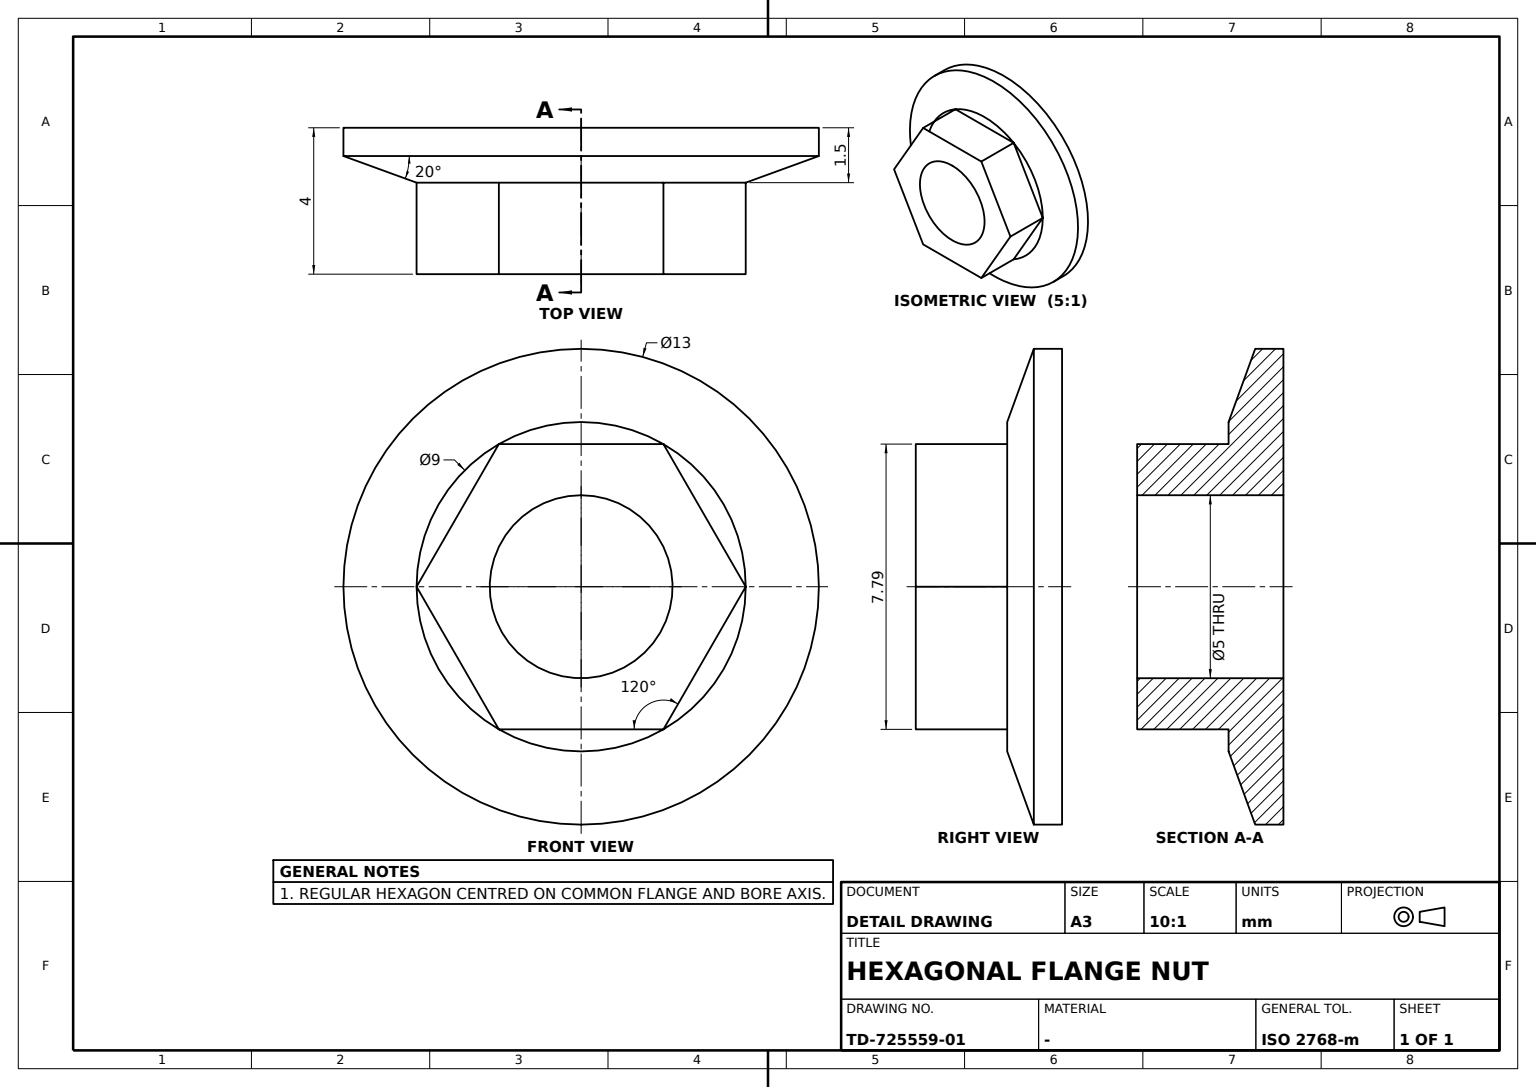
ISO-10303-21;
HEADER;
FILE_DESCRIPTION((''),'2;1');
FILE_NAME('','',(''),(''),'','','');
FILE_SCHEMA(('AUTOMOTIVE_DESIGN'));
ENDSEC;
DATA;
#1=APPLICATION_CONTEXT('');
#2=PRODUCT_CONTEXT('',#1,'mechanical');
#3=PRODUCT('','','',(#2));
#4=PRODUCT_DEFINITION_FORMATION('','',#3);
#5=PRODUCT_DEFINITION_CONTEXT('',#1,'design');
#6=PRODUCT_DEFINITION('','',#4,#5);
#7=PRODUCT_DEFINITION_SHAPE('','',#6);
#8=(LENGTH_UNIT()NAMED_UNIT(*)SI_UNIT(.MILLI.,.METRE.));
#9=(NAMED_UNIT(*)PLANE_ANGLE_UNIT()SI_UNIT($,.RADIAN.));
#10=(NAMED_UNIT(*)SI_UNIT($,.STERADIAN.)SOLID_ANGLE_UNIT());
#11=UNCERTAINTY_MEASURE_WITH_UNIT(LENGTH_MEASURE(0.005),#8,'distance_accuracy_value','');
#12=(GEOMETRIC_REPRESENTATION_CONTEXT(3)GLOBAL_UNCERTAINTY_ASSIGNED_CONTEXT((#11))GLOBAL_UNIT_ASSIGNED_CONTEXT((#8,#9,#10))REPRESENTATION_CONTEXT('',''));
#13=CARTESIAN_POINT('',(-1.5,4.5,0.));
#14=VERTEX_POINT('',#13);
#15=CARTESIAN_POINT('',(-1.5,2.25,3.897114));
#16=VERTEX_POINT('',#15);
#17=CARTESIAN_POINT('',(-1.5,0.,0.));
#18=DIRECTION('',(1.,0.,0.));
#19=DIRECTION('',(0.,0.,-1.));
#20=AXIS2_PLACEMENT_3D('',#17,#18,#19);
#21=CIRCLE('',#20,4.5);
#22=EDGE_CURVE('',#14,#16,#21,.T.);
#23=ORIENTED_EDGE('',*,*,#22,.F.);
#24=DIRECTION('',(0.,0.5,-0.866025404));
#25=VECTOR('',#24,1000.);
#26=LINE('',#15,#25);
#27=EDGE_CURVE('',#16,#14,#26,.T.);
#28=ORIENTED_EDGE('',*,*,#27,.F.);
#29=EDGE_LOOP('',(#23,#28));
#30=FACE_BOUND('',#29,.T.);
#31=DIRECTION('',(0.,1.,0.));
#32=AXIS2_PLACEMENT_3D('',#13,#18,#31);
#33=PLANE('',#32);
#34=ADVANCED_FACE('',(#30),#33,.F.);
#35=CARTESIAN_POINT('',(-0.77206,0.,-6.5));
#36=VERTEX_POINT('',#35);
#37=CARTESIAN_POINT('',(-0.77206,0.,0.));
#38=AXIS2_PLACEMENT_3D('',#37,#18,#19);
#39=CIRCLE('',#38,6.5);
#40=EDGE_CURVE('',#36,#36,#39,.T.);
#41=ORIENTED_EDGE('',*,*,#40,.F.);
#42=EDGE_LOOP('',(#41));
#43=FACE_BOUND('',#42,.T.);
#44=CARTESIAN_POINT('',(-1.5,-2.25,3.897114));
#45=VERTEX_POINT('',#44);
#46=EDGE_CURVE('',#16,#45,#21,.T.);
#47=ORIENTED_EDGE('',*,*,#46,.T.);
#48=CARTESIAN_POINT('',(-1.5,-4.5,0.));
#49=VERTEX_POINT('',#48);
#50=EDGE_CURVE('',#45,#49,#21,.T.);
#51=ORIENTED_EDGE('',*,*,#50,.T.);
#52=CARTESIAN_POINT('',(-1.5,-2.25,-3.897114));
#53=VERTEX_POINT('',#52);
#54=EDGE_CURVE('',#49,#53,#21,.T.);
#55=ORIENTED_EDGE('',*,*,#54,.T.);
#56=CARTESIAN_POINT('',(-1.5,2.25,-3.897114));
#57=VERTEX_POINT('',#56);
#58=EDGE_CURVE('',#53,#57,#21,.T.);
#59=ORIENTED_EDGE('',*,*,#58,.T.);
#60=EDGE_CURVE('',#57,#14,#21,.T.);
#61=ORIENTED_EDGE('',*,*,#60,.T.);
#62=ORIENTED_EDGE('',*,*,#22,.T.);
#63=EDGE_LOOP('',(#47,#51,#55,#59,#61,#62));
#64=FACE_BOUND('',#63,.T.);
#65=AXIS2_PLACEMENT_3D('',#17,#18,#31);
#66=CONICAL_SURFACE('',#65,4.5,1.221730476);
#67=ADVANCED_FACE('',(#43,#64),#66,.T.);
#68=CARTESIAN_POINT('',(-4.,-4.5,0.));
#69=VERTEX_POINT('',#68);
#70=CARTESIAN_POINT('',(-4.,-2.25,3.897114));
#71=VERTEX_POINT('',#70);
#72=CARTESIAN_POINT('',(-4.,-3.375,1.948557));
#73=DIRECTION('',(0.,0.5,0.866025404));
#74=VECTOR('',#73,1000.);
#75=LINE('',#72,#74);
#76=EDGE_CURVE('',#69,#71,#75,.T.);
#77=ORIENTED_EDGE('',*,*,#76,.T.);
#78=CARTESIAN_POINT('',(-4.,2.25,3.897114));
#79=VERTEX_POINT('',#78);
#80=CARTESIAN_POINT('',(-4.,0.,3.897114));
#81=VECTOR('',#31,1000.);
#82=LINE('',#80,#81);
#83=EDGE_CURVE('',#71,#79,#82,.T.);
#84=ORIENTED_EDGE('',*,*,#83,.T.);
#85=CARTESIAN_POINT('',(-4.,4.5,0.));
#86=VERTEX_POINT('',#85);
#87=CARTESIAN_POINT('',(-4.,3.375,1.948557));
#88=LINE('',#87,#25);
#89=EDGE_CURVE('',#79,#86,#88,.T.);
#90=ORIENTED_EDGE('',*,*,#89,.T.);
#91=CARTESIAN_POINT('',(-4.,2.25,-3.897114));
#92=VERTEX_POINT('',#91);
#93=CARTESIAN_POINT('',(-4.,3.375,-1.948557));
#94=DIRECTION('',(0.,-0.5,-0.866025404));
#95=VECTOR('',#94,1000.);
#96=LINE('',#93,#95);
#97=EDGE_CURVE('',#86,#92,#96,.T.);
#98=ORIENTED_EDGE('',*,*,#97,.T.);
#99=CARTESIAN_POINT('',(-4.,-2.25,-3.897114));
#100=VERTEX_POINT('',#99);
#101=CARTESIAN_POINT('',(-4.,0.,-3.897114));
#102=DIRECTION('',(0.,-1.,0.));
#103=VECTOR('',#102,1000.);
#104=LINE('',#101,#103);
#105=EDGE_CURVE('',#92,#100,#104,.T.);
#106=ORIENTED_EDGE('',*,*,#105,.T.);
#107=CARTESIAN_POINT('',(-4.,-3.375,-1.948557));
#108=DIRECTION('',(0.,-0.5,0.866025404));
#109=VECTOR('',#108,1000.);
#110=LINE('',#107,#109);
#111=EDGE_CURVE('',#100,#69,#110,.T.);
#112=ORIENTED_EDGE('',*,*,#111,.T.);
#113=EDGE_LOOP('',(#77,#84,#90,#98,#106,#112));
#114=FACE_BOUND('',#113,.T.);
#115=CARTESIAN_POINT('',(-4.,0.,2.5));
#116=VERTEX_POINT('',#115);
#117=CARTESIAN_POINT('',(-4.,0.,0.));
#118=DIRECTION('',(-1.,0.,0.));
#119=DIRECTION('',(0.,0.,1.));
#120=AXIS2_PLACEMENT_3D('',#117,#118,#119);
#121=CIRCLE('',#120,2.5);
#122=EDGE_CURVE('',#116,#116,#121,.T.);
#123=ORIENTED_EDGE('',*,*,#122,.F.);
#124=EDGE_LOOP('',(#123));
#125=FACE_BOUND('',#124,.T.);
#126=AXIS2_PLACEMENT_3D('',#117,#118,#102);
#127=PLANE('',#126);
#128=ADVANCED_FACE('',(#114,#125),#127,.T.);
#129=VECTOR('',#118,1000.);
#130=LINE('',#48,#129);
#131=EDGE_CURVE('',#49,#69,#130,.T.);
#132=ORIENTED_EDGE('',*,*,#131,.F.);
#133=LINE('',#48,#74);
#134=EDGE_CURVE('',#49,#45,#133,.T.);
#135=ORIENTED_EDGE('',*,*,#134,.T.);
#136=LINE('',#44,#129);
#137=EDGE_CURVE('',#45,#71,#136,.T.);
#138=ORIENTED_EDGE('',*,*,#137,.T.);
#139=ORIENTED_EDGE('',*,*,#76,.F.);
#140=EDGE_LOOP('',(#132,#135,#138,#139));
#141=FACE_BOUND('',#140,.T.);
#142=DIRECTION('',(0.,-0.866025404,0.5));
#143=AXIS2_PLACEMENT_3D('',#48,#142,#73);
#144=PLANE('',#143);
#145=ADVANCED_FACE('',(#141),#144,.T.);
#146=ORIENTED_EDGE('',*,*,#83,.F.);
#147=ORIENTED_EDGE('',*,*,#137,.F.);
#148=LINE('',#44,#81);
#149=EDGE_CURVE('',#45,#16,#148,.T.);
#150=ORIENTED_EDGE('',*,*,#149,.T.);
#151=LINE('',#15,#129);
#152=EDGE_CURVE('',#16,#79,#151,.T.);
#153=ORIENTED_EDGE('',*,*,#152,.T.);
#154=EDGE_LOOP('',(#146,#147,#150,#153));
#155=FACE_BOUND('',#154,.T.);
#156=AXIS2_PLACEMENT_3D('',#44,#119,#31);
#157=PLANE('',#156);
#158=ADVANCED_FACE('',(#155),#157,.T.);
#159=ORIENTED_EDGE('',*,*,#122,.T.);
#160=EDGE_LOOP('',(#159));
#161=FACE_BOUND('',#160,.T.);
#162=CARTESIAN_POINT('',(0.,0.,-2.5));
#163=VERTEX_POINT('',#162);
#164=CARTESIAN_POINT('',(0.,0.,0.));
#165=AXIS2_PLACEMENT_3D('',#164,#18,#19);
#166=CIRCLE('',#165,2.5);
#167=EDGE_CURVE('',#163,#163,#166,.T.);
#168=ORIENTED_EDGE('',*,*,#167,.T.);
#169=EDGE_LOOP('',(#168));
#170=FACE_BOUND('',#169,.T.);
#171=CARTESIAN_POINT('',(-1.34,0.,0.));
#172=AXIS2_PLACEMENT_3D('',#171,#118,#102);
#173=CYLINDRICAL_SURFACE('',#172,2.5);
#174=ADVANCED_FACE('',(#161,#170),#173,.F.);
#175=ORIENTED_EDGE('',*,*,#111,.F.);
#176=LINE('',#52,#129);
#177=EDGE_CURVE('',#53,#100,#176,.T.);
#178=ORIENTED_EDGE('',*,*,#177,.F.);
#179=LINE('',#52,#109);
#180=EDGE_CURVE('',#53,#49,#179,.T.);
#181=ORIENTED_EDGE('',*,*,#180,.T.);
#182=ORIENTED_EDGE('',*,*,#131,.T.);
#183=EDGE_LOOP('',(#175,#178,#181,#182));
#184=FACE_BOUND('',#183,.T.);
#185=DIRECTION('',(0.,-0.866025404,-0.5));
#186=AXIS2_PLACEMENT_3D('',#52,#185,#108);
#187=PLANE('',#186);
#188=ADVANCED_FACE('',(#184),#187,.T.);
#189=ORIENTED_EDGE('',*,*,#54,.F.);
#190=ORIENTED_EDGE('',*,*,#180,.F.);
#191=EDGE_LOOP('',(#189,#190));
#192=FACE_BOUND('',#191,.T.);
#193=ADVANCED_FACE('',(#192),#33,.F.);
#194=ORIENTED_EDGE('',*,*,#58,.F.);
#195=LINE('',#56,#103);
#196=EDGE_CURVE('',#57,#53,#195,.T.);
#197=ORIENTED_EDGE('',*,*,#196,.F.);
#198=EDGE_LOOP('',(#194,#197));
#199=FACE_BOUND('',#198,.T.);
#200=ADVANCED_FACE('',(#199),#33,.F.);
#201=ORIENTED_EDGE('',*,*,#152,.F.);
#202=ORIENTED_EDGE('',*,*,#27,.T.);
#203=LINE('',#13,#129);
#204=EDGE_CURVE('',#14,#86,#203,.T.);
#205=ORIENTED_EDGE('',*,*,#204,.T.);
#206=ORIENTED_EDGE('',*,*,#89,.F.);
#207=EDGE_LOOP('',(#201,#202,#205,#206));
#208=FACE_BOUND('',#207,.T.);
#209=DIRECTION('',(0.,0.866025404,0.5));
#210=AXIS2_PLACEMENT_3D('',#15,#209,#24);
#211=PLANE('',#210);
#212=ADVANCED_FACE('',(#208),#211,.T.);
#213=ORIENTED_EDGE('',*,*,#50,.F.);
#214=ORIENTED_EDGE('',*,*,#134,.F.);
#215=EDGE_LOOP('',(#213,#214));
#216=FACE_BOUND('',#215,.T.);
#217=ADVANCED_FACE('',(#216),#33,.F.);
#218=ORIENTED_EDGE('',*,*,#60,.F.);
#219=LINE('',#13,#95);
#220=EDGE_CURVE('',#14,#57,#219,.T.);
#221=ORIENTED_EDGE('',*,*,#220,.F.);
#222=EDGE_LOOP('',(#218,#221));
#223=FACE_BOUND('',#222,.T.);
#224=ADVANCED_FACE('',(#223),#33,.F.);
#225=ORIENTED_EDGE('',*,*,#196,.T.);
#226=ORIENTED_EDGE('',*,*,#177,.T.);
#227=ORIENTED_EDGE('',*,*,#105,.F.);
#228=LINE('',#56,#129);
#229=EDGE_CURVE('',#57,#92,#228,.T.);
#230=ORIENTED_EDGE('',*,*,#229,.F.);
#231=EDGE_LOOP('',(#225,#226,#227,#230));
#232=FACE_BOUND('',#231,.T.);
#233=AXIS2_PLACEMENT_3D('',#56,#19,#102);
#234=PLANE('',#233);
#235=ADVANCED_FACE('',(#232),#234,.T.);
#236=ORIENTED_EDGE('',*,*,#220,.T.);
#237=ORIENTED_EDGE('',*,*,#229,.T.);
#238=ORIENTED_EDGE('',*,*,#97,.F.);
#239=ORIENTED_EDGE('',*,*,#204,.F.);
#240=EDGE_LOOP('',(#236,#237,#238,#239));
#241=FACE_BOUND('',#240,.T.);
#242=DIRECTION('',(0.,0.866025404,-0.5));
#243=AXIS2_PLACEMENT_3D('',#13,#242,#94);
#244=PLANE('',#243);
#245=ADVANCED_FACE('',(#241),#244,.T.);
#246=ORIENTED_EDGE('',*,*,#46,.F.);
#247=ORIENTED_EDGE('',*,*,#149,.F.);
#248=EDGE_LOOP('',(#246,#247));
#249=FACE_BOUND('',#248,.T.);
#250=ADVANCED_FACE('',(#249),#33,.F.);
#251=CARTESIAN_POINT('',(0.,0.,-6.5));
#252=VERTEX_POINT('',#251);
#253=CIRCLE('',#165,6.5);
#254=EDGE_CURVE('',#252,#252,#253,.T.);
#255=ORIENTED_EDGE('',*,*,#254,.F.);
#256=EDGE_LOOP('',(#255));
#257=FACE_BOUND('',#256,.T.);
#258=ORIENTED_EDGE('',*,*,#40,.T.);
#259=EDGE_LOOP('',(#258));
#260=FACE_BOUND('',#259,.T.);
#261=CARTESIAN_POINT('',(-0.75,0.,0.));
#262=AXIS2_PLACEMENT_3D('',#261,#18,#31);
#263=CYLINDRICAL_SURFACE('',#262,6.5);
#264=ADVANCED_FACE('',(#257,#260),#263,.T.);
#265=ORIENTED_EDGE('',*,*,#254,.T.);
#266=EDGE_LOOP('',(#265));
#267=FACE_BOUND('',#266,.T.);
#268=ORIENTED_EDGE('',*,*,#167,.F.);
#269=EDGE_LOOP('',(#268));
#270=FACE_BOUND('',#269,.T.);
#271=AXIS2_PLACEMENT_3D('',#164,#18,#31);
#272=PLANE('',#271);
#273=ADVANCED_FACE('',(#267,#270),#272,.T.);
#274=CLOSED_SHELL('',(#34,#67,#128,#145,#158,#174,#188,#193,#200,#212,#217,#224,#235,#245,#250,#264,#273));
#275=MANIFOLD_SOLID_BREP('',#274);
#276=ADVANCED_BREP_SHAPE_REPRESENTATION('',(#275),#12);
#277=SHAPE_DEFINITION_REPRESENTATION(#7,#276);
ENDSEC;
END-ISO-10303-21;
